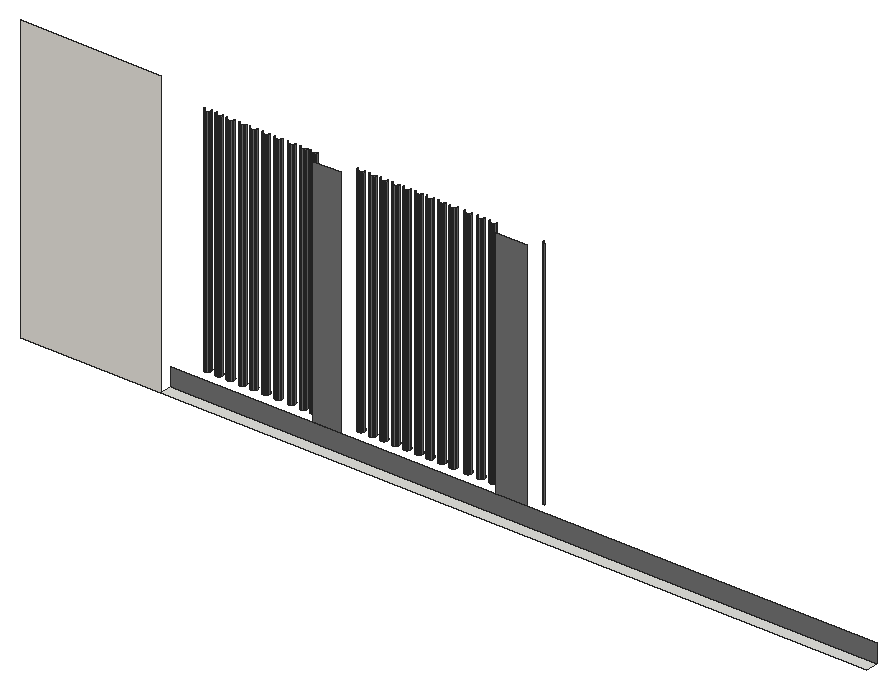
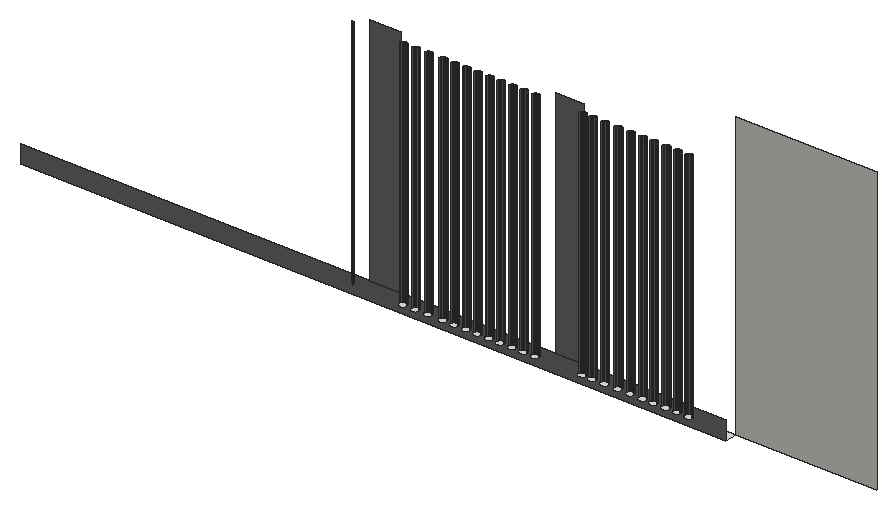
# SketchUp Ruby script. Lengths in inches.
U = 1.inch
M = Sketchup.active_model
def pt(a) = Geom::Point3d.new(a.map { |v| v * U })
def face(e, loops, mat)
  f = e.add_face(loops[0].map { |a| pt(a) })
  loops[1..].each { |l| e.add_face(l.map { |a| pt(a) }).erase! }
  f.material = f.back_material = mat if mat
  f
end
# faces: each face lists its corners as indices into pts; further lists are holes
def faces(e, pts, list, mat = nil) = list.each { |f| face(e, (f[0].is_a?(Array) ? f : [f]).map { |l| l.map { |i| pts[i] } }, mat) }
# xy, xz, yz: faces in a plane at the given z, y or x. An outline is a flat list of corners, or four numbers for a rectangle; further outlines are holes
def ring(l) = l.size == 4 ? [[l[0], l[1]], [l[2], l[1]], [l[2], l[3]], [l[0], l[3]]] : l.each_slice(2).to_a
def flat(e, list, mat, &to3) = list.each { |f| face(e, (f[0].is_a?(Array) ? f : [f]).map { |l| ring(l).map { |u, v| to3.(u, v) } }, mat) }
def xy(e, z, list, mat = nil) = flat(e, list, mat) { |x, y| [x, y, z] }
def xz(e, y, list, mat = nil) = flat(e, list, mat) { |x, z| [x, y, z] }
def yz(e, x, list, mat = nil) = flat(e, list, mat) { |y, z| [x, y, z] }
def lines(e, pts, list) = list.each { |a, b| e.add_line(pt(pts[a]), pt(pts[b])) }
# prism: a flat outline (further loops are holes) pulled along v
def prism(e, loops, v, mat = nil)
  f = face(e, loops, mat); d = Geom::Vector3d.new(v.map { |x| x * U })
  f.pushpull(f.normal.samedirection?(d) ? d.length : -d.length)
end
def box(e, o, s, mat = nil) = prism(e, [[o, [o[0] + s[0], o[1], o[2]], [o[0] + s[0], o[1] + s[1], o[2]], [o[0], o[1] + s[1], o[2]]]], [0, 0, s[2]], mat)
def at(x, y, z, deg = 0) = Geom::Transformation.translation(pt([x, y, z])) * Geom::Transformation.rotation(ORIGIN, Z_AXIS, deg.degrees)
def axes(o, x, y, z) = Geom::Transformation.new([*x, 0, *y, 0, *z, 0, *pt(o).to_a, 1])
def part(name) = M.definitions.add(name)
# library, detail: a bought-in or finely detailed component or shape, given as its bounding box
def library(name, o, s) = part(name).tap { |d| box(d.entities, o, s) }
def detail(e, o, s) = box(e.add_group.entities, o, s)
def put(e, d, t, mat = nil) = e.add_instance(d, t).tap { |i| i.material = mat if mat }
def group(e, t, mat = nil) = e.add_group.tap { |g| g.transformation = t; g.material = mat if mat }.entities
root = M.entities
M.materials.add("[Color M05]").color = [114, 114, 114]
M.materials.add("[Tile Travertine 2 inch]").color = [229, 225, 218]
xy(root,9,[[61.88,119.71,371.37,125.1875]])
xy(root,17.125,[[73.24,129.51,72.84,129.56,72.46,129.72,72.13,129.97,71.89,130.29,71.73,130.67,71.68,131.07,71.73,131.48,71.89,131.86,72.13,132.18,72.46,132.43,72.84,132.58,73.24,132.64,73.64,132.58,74.02,132.43,74.34,132.18,74.59,131.86,74.75,131.48,74.8,131.07,74.75,130.67,74.59,130.29,74.34,129.97,74.02,129.72,73.64,129.56],[78.3,129.51,77.9,129.56,77.52,129.72,77.2,129.97,76.95,130.29,76.79,130.67,76.74,131.07,76.79,131.48,76.95,131.86,77.2,132.18,77.52,132.43,77.9,132.58,78.3,132.64,78.71,132.58,79.08,132.43,79.41,132.18,79.66,131.86,79.8125,131.48,79.86,131.07,79.8125,130.67,79.66,130.29,79.41,129.97,79.08,129.72,78.71,129.56],[83.3,129.51,82.9,129.56,82.52,129.72,82.2,129.97,81.95,130.29,81.79,130.67,81.74,131.07,81.79,131.48,81.95,131.86,82.2,132.18,82.52,132.43,82.9,132.58,83.3,132.64,83.71,132.58,84.08,132.43,84.41,132.18,84.66,131.86,84.8125,131.48,84.86,131.07,84.8125,130.67,84.66,130.29,84.41,129.97,84.08,129.72,83.71,129.56],[88.61,129.51,88.21,129.56,87.83,129.72,87.51,129.97,87.26,130.29,87.11,130.67,87.05,131.07,87.11,131.48,87.26,131.86,87.51,132.18,87.83,132.43,88.21,132.58,88.61,132.64,89.02,132.58,89.4,132.43,89.72,132.18,89.97,131.86,90.125,131.48,90.18,131.07,90.125,130.67,89.97,130.29,89.72,129.97,89.4,129.72,89.02,129.56],[93.43,129.51,93.02,129.56,92.65,129.72,92.32,129.97,92.07,130.29,91.92,130.67,91.86,131.07,91.92,131.48,92.07,131.86,92.32,132.18,92.65,132.43,93.02,132.58,93.43,132.64,93.83,132.58,94.21,132.43,94.53,132.18,94.78,131.86,94.9375,131.48,94.99,131.07,94.9375,130.67,94.78,130.29,94.53,129.97,94.21,129.72,93.83,129.56],
  [98.93,129.51,98.52,129.56,98.15,129.72,97.82,129.97,97.57,130.29,97.42,130.67,97.36,131.07,97.42,131.48,97.57,131.86,97.82,132.18,98.15,132.43,98.52,132.58,98.93,132.64,99.33,132.58,99.71,132.43,100.03,132.18,100.28,131.86,100.4375,131.48,100.49,131.07,100.4375,130.67,100.28,130.29,100.03,129.97,99.71,129.72,99.33,129.56],[104.36,129.51,103.96,129.56,103.58,129.72,103.26,129.97,103.01,130.29,102.86,130.67,102.8,131.07,102.86,131.48,103.01,131.86,103.26,132.18,103.58,132.43,103.96,132.58,104.36,132.64,104.77,132.58,105.15,132.43,105.47,132.18,105.72,131.86,105.875,131.48,105.93,131.07,105.875,130.67,105.72,130.29,105.47,129.97,105.15,129.72,104.77,129.56],[110.11,129.51,109.71,129.56,109.33,129.72,109.01,129.97,108.76,130.29,108.61,130.67,108.55,131.07,108.61,131.48,108.76,131.86,109.01,132.18,109.33,132.43,109.71,132.58,110.11,132.64,110.52,132.58,110.9,132.43,111.22,132.18,111.47,131.86,111.625,131.48,111.68,131.07,111.625,130.67,111.47,130.29,111.22,129.97,110.9,129.72,110.52,129.56],[115.49,129.51,115.09,129.56,114.71,129.72,114.38,129.97,114.14,130.29,113.98,130.67,113.93,131.07,113.98,131.48,114.14,131.86,114.38,132.18,114.71,132.43,115.09,132.58,115.49,132.64,115.89,132.58,116.27,132.43,116.59,132.18,116.84,131.86,117,131.48,117.05,131.07,117,130.67,116.84,130.29,116.59,129.97,116.27,129.72,115.89,129.56],[119.99,129.51,119.59,129.56,119.21,129.72,118.88,129.97,118.64,130.29,118.48,130.67,118.43,131.07,118.48,131.48,118.64,131.86,118.88,132.18,119.21,132.43,119.59,132.58,119.99,132.64,120.39,132.58,120.77,132.43,121.09,132.18,121.34,131.86,121.5,131.48,121.55,131.07,121.5,130.67,121.34,130.29,121.09,129.97,120.77,129.72,120.39,129.56],
  [140.68,129.51,140.27,129.56,139.9,129.72,139.57,129.97,139.32,130.29,139.17,130.67,139.11,131.07,139.17,131.48,139.32,131.86,139.57,132.18,139.9,132.43,140.27,132.58,140.68,132.64,141.08,132.58,141.46,132.43,141.78,132.18,142.03,131.86,142.1875,131.48,142.24,131.07,142.1875,130.67,142.03,130.29,141.78,129.97,141.46,129.72,141.08,129.56],[145.74,129.51,145.34,129.56,144.96,129.72,144.63,129.97,144.39,130.29,144.23,130.67,144.18,131.07,144.23,131.48,144.39,131.86,144.63,132.18,144.96,132.43,145.34,132.58,145.74,132.64,146.14,132.58,146.52,132.43,146.84,132.18,147.09,131.86,147.25,131.48,147.3,131.07,147.25,130.67,147.09,130.29,146.84,129.97,146.52,129.72,146.14,129.56],[150.8,129.51,150.4,129.56,150.02,129.72,149.7,129.97,149.45,130.29,149.29,130.67,149.24,131.07,149.29,131.48,149.45,131.86,149.7,132.18,150.02,132.43,150.4,132.58,150.8,132.64,151.21,132.58,151.58,132.43,151.91,132.18,152.16,131.86,152.3125,131.48,152.36,131.07,152.3125,130.67,152.16,130.29,151.91,129.97,151.58,129.72,151.21,129.56],[155.86,129.51,155.46,129.56,155.08,129.72,154.76,129.97,154.51,130.29,154.36,130.67,154.3,131.07,154.36,131.48,154.51,131.86,154.76,132.18,155.08,132.43,155.46,132.58,155.86,132.64,156.27,132.58,156.65,132.43,156.97,132.18,157.22,131.86,157.375,131.48,157.43,131.07,157.375,130.67,157.22,130.29,156.97,129.97,156.65,129.72,156.27,129.56],[160.93,129.51,160.52,129.56,160.15,129.72,159.82,129.97,159.57,130.29,159.42,130.67,159.36,131.07,159.42,131.48,159.57,131.86,159.82,132.18,160.15,132.43,160.52,132.58,160.93,132.64,161.33,132.58,161.71,132.43,162.03,132.18,162.28,131.86,162.4375,131.48,162.49,131.07,162.4375,130.67,162.28,130.29,162.03,129.97,161.71,129.72,161.33,129.56],
  [165.99,129.51,165.59,129.56,165.21,129.72,164.88,129.97,164.64,130.29,164.48,130.67,164.43,131.07,164.48,131.48,164.64,131.86,164.88,132.18,165.21,132.43,165.59,132.58,165.99,132.64,166.39,132.58,166.77,132.43,167.09,132.18,167.34,131.86,167.5,131.48,167.55,131.07,167.5,130.67,167.34,130.29,167.09,129.97,166.77,129.72,166.39,129.56],[171.05,129.51,170.65,129.56,170.27,129.72,169.95,129.97,169.7,130.29,169.54,130.67,169.49,131.07,169.54,131.48,169.7,131.86,169.95,132.18,170.27,132.43,170.65,132.58,171.05,132.64,171.46,132.58,171.83,132.43,172.16,132.18,172.41,131.86,172.5625,131.48,172.61,131.07,172.5625,130.67,172.41,130.29,172.16,129.97,171.83,129.72,171.46,129.56],[176.11,129.51,175.71,129.56,175.33,129.72,175.01,129.97,174.76,130.29,174.61,130.67,174.55,131.07,174.61,131.48,174.76,131.86,175.01,132.18,175.33,132.43,175.71,132.58,176.11,132.64,176.52,132.58,176.9,132.43,177.22,132.18,177.47,131.86,177.625,131.48,177.68,131.07,177.625,130.67,177.47,130.29,177.22,129.97,176.9,129.72,176.52,129.56],[181.18,129.51,180.77,129.56,180.4,129.72,180.07,129.97,179.82,130.29,179.67,130.67,179.61,131.07,179.67,131.48,179.82,131.86,180.07,132.18,180.4,132.43,180.77,132.58,181.18,132.64,181.58,132.58,181.96,132.43,182.28,132.18,182.53,131.86,182.6875,131.48,182.74,131.07,182.6875,130.67,182.53,130.29,182.28,129.97,181.96,129.72,181.58,129.56],[187.68,129.51,187.27,129.56,186.9,129.72,186.57,129.97,186.32,130.29,186.17,130.67,186.11,131.07,186.17,131.48,186.32,131.86,186.57,132.18,186.9,132.43,187.27,132.58,187.68,132.64,188.08,132.58,188.46,132.43,188.78,132.18,189.03,131.86,189.1875,131.48,189.24,131.07,189.1875,130.67,189.03,130.29,188.78,129.97,188.46,129.72,188.08,129.56],
  [193.18,129.51,192.77,129.56,192.4,129.72,192.07,129.97,191.82,130.29,191.67,130.67,191.61,131.07,191.67,131.48,191.82,131.86,192.07,132.18,192.4,132.43,192.77,132.58,193.18,132.64,193.58,132.58,193.96,132.43,194.28,132.18,194.53,131.86,194.6875,131.48,194.74,131.07,194.6875,130.67,194.53,130.29,194.28,129.97,193.96,129.72,193.58,129.56],[198.68,129.51,198.27,129.56,197.9,129.72,197.57,129.97,197.32,130.29,197.17,130.67,197.11,131.07,197.17,131.48,197.32,131.86,197.57,132.18,197.9,132.43,198.27,132.58,198.68,132.64,199.08,132.58,199.46,132.43,199.78,132.18,200.03,131.86,200.1875,131.48,200.24,131.07,200.1875,130.67,200.03,130.29,199.78,129.97,199.46,129.72,199.08,129.56]])
xz(root,119.71,[[0,9,61.88,133.9375]],"[Tile Travertine 2 inch]")
xz(root,125.1875,[[61.88,9,371.37,17.125],[124.17,17.125,136.24,119.59],[204.36,17.125,217.93,119.59]],"[Color M05]")
p = [[72.84,129.56,17.125],[73.24,129.51,17.125],[73.24,129.51,119.59],[72.84,129.56,119.59],[73.64,129.56,17.125],[73.64,129.56,119.59],
  [77.9,129.56,17.125],[78.3,129.51,17.125],[78.3,129.51,119.59],[77.9,129.56,119.59],[78.71,129.56,17.125],[78.71,129.56,119.59],
  [82.9,129.56,17.125],[83.3,129.51,17.125],[83.3,129.51,119.59],[82.9,129.56,119.59],[83.71,129.56,17.125],[83.71,129.56,119.59],
  [88.21,129.56,17.125],[88.61,129.51,17.125],[88.61,129.51,119.59],[88.21,129.56,119.59],[89.02,129.56,17.125],[89.02,129.56,119.59],
  [93.02,129.56,17.125],[93.43,129.51,17.125],[93.43,129.51,119.59],[93.02,129.56,119.59],[93.83,129.56,17.125],[93.83,129.56,119.59],
  [98.52,129.56,17.125],[98.93,129.51,17.125],[98.93,129.51,119.59],[98.52,129.56,119.59],[99.33,129.56,17.125],[99.33,129.56,119.59],
  [103.96,129.56,17.125],[104.36,129.51,17.125],[104.36,129.51,119.59],[103.96,129.56,119.59],[104.77,129.56,17.125],[104.77,129.56,119.59],
  [109.71,129.56,17.125],[110.11,129.51,17.125],[110.11,129.51,119.59],[109.71,129.56,119.59],[110.52,129.56,17.125],[110.52,129.56,119.59],
  [115.09,129.56,17.125],[115.49,129.51,17.125],[115.49,129.51,119.59],[115.09,129.56,119.59],[115.89,129.56,17.125],[115.89,129.56,119.59],
  [119.59,129.56,17.125],[119.99,129.51,17.125],[119.99,129.51,119.59],[119.59,129.56,119.59],[120.39,129.56,17.125],[120.39,129.56,119.59],
  [140.27,129.56,17.125],[140.68,129.51,17.125],[140.68,129.51,119.59],[140.27,129.56,119.59],[141.08,129.56,17.125],[141.08,129.56,119.59],
  [145.34,129.56,17.125],[145.74,129.51,17.125],[145.74,129.51,119.59],[145.34,129.56,119.59],[146.14,129.56,17.125],[146.14,129.56,119.59],
  [150.4,129.56,17.125],[150.8,129.51,17.125],[150.8,129.51,119.59],[150.4,129.56,119.59],[151.21,129.56,17.125],[151.21,129.56,119.59],
  [155.46,129.56,17.125],[155.86,129.51,17.125],[155.86,129.51,119.59],[155.46,129.56,119.59],[156.27,129.56,17.125],[156.27,129.56,119.59],
  [160.52,129.56,17.125],[160.93,129.51,17.125],[160.93,129.51,119.59],[160.52,129.56,119.59],[161.33,129.56,17.125],[161.33,129.56,119.59],
  [165.59,129.56,17.125],[165.99,129.51,17.125],[165.99,129.51,119.59],[165.59,129.56,119.59],[166.39,129.56,17.125],[166.39,129.56,119.59],
  [170.65,129.56,17.125],[171.05,129.51,17.125],[171.05,129.51,119.59],[170.65,129.56,119.59],[171.46,129.56,17.125],[171.46,129.56,119.59],
  [175.71,129.56,17.125],[176.11,129.51,17.125],[176.11,129.51,119.59],[175.71,129.56,119.59],[176.52,129.56,17.125],[176.52,129.56,119.59],
  [180.77,129.56,17.125],[181.18,129.51,17.125],[181.18,129.51,119.59],[180.77,129.56,119.59],[181.58,129.56,17.125],[181.58,129.56,119.59],
  [187.27,129.56,17.125],[187.68,129.51,17.125],[187.68,129.51,119.59],[187.27,129.56,119.59],[188.08,129.56,17.125],[188.08,129.56,119.59],
  [192.77,129.56,17.125],[193.18,129.51,17.125],[193.18,129.51,119.59],[192.77,129.56,119.59],[193.58,129.56,17.125],[193.58,129.56,119.59],
  [198.27,129.56,17.125],[198.68,129.51,17.125],[198.68,129.51,119.59],[198.27,129.56,119.59],[199.08,129.56,17.125],[199.08,129.56,119.59],
  [221.84,129.56,17.125],[222.24,129.51,17.125],[222.24,129.51,119.59],[221.84,129.56,119.59],[72.46,129.72,17.125],[72.46,129.72,119.59],
  [74.02,129.72,17.125],[74.02,129.72,119.59],[77.52,129.72,17.125],[77.52,129.72,119.59],[79.08,129.72,17.125],[79.08,129.72,119.59],
  [82.52,129.72,17.125],[82.52,129.72,119.59],[84.08,129.72,17.125],[84.08,129.72,119.59],[87.83,129.72,17.125],[87.83,129.72,119.59],
  [89.4,129.72,17.125],[89.4,129.72,119.59],[92.65,129.72,17.125],[92.65,129.72,119.59],[94.21,129.72,17.125],[94.21,129.72,119.59],
  [98.15,129.72,17.125],[98.15,129.72,119.59],[99.71,129.72,17.125],[99.71,129.72,119.59],[103.58,129.72,17.125],[103.58,129.72,119.59],
  [105.15,129.72,17.125],[105.15,129.72,119.59],[109.33,129.72,17.125],[109.33,129.72,119.59],[110.9,129.72,17.125],[110.9,129.72,119.59],
  [114.71,129.72,17.125],[114.71,129.72,119.59],[116.27,129.72,17.125],[116.27,129.72,119.59],[119.21,129.72,17.125],[119.21,129.72,119.59],
  [120.77,129.72,17.125],[120.77,129.72,119.59],[139.9,129.72,17.125],[139.9,129.72,119.59],[141.46,129.72,17.125],[141.46,129.72,119.59],
  [144.96,129.72,17.125],[144.96,129.72,119.59],[146.52,129.72,17.125],[146.52,129.72,119.59],[150.02,129.72,17.125],[150.02,129.72,119.59],
  [151.58,129.72,17.125],[151.58,129.72,119.59],[155.08,129.72,17.125],[155.08,129.72,119.59],[156.65,129.72,17.125],[156.65,129.72,119.59],
  [160.15,129.72,17.125],[160.15,129.72,119.59],[161.71,129.72,17.125],[161.71,129.72,119.59],[165.21,129.72,17.125],[165.21,129.72,119.59],
  [166.77,129.72,17.125],[166.77,129.72,119.59],[170.27,129.72,17.125],[170.27,129.72,119.59],[171.83,129.72,17.125],[171.83,129.72,119.59],
  [175.33,129.72,17.125],[175.33,129.72,119.59],[176.9,129.72,17.125],[176.9,129.72,119.59],[180.4,129.72,17.125],[180.4,129.72,119.59],
  [181.96,129.72,17.125],[181.96,129.72,119.59],[186.9,129.72,17.125],[186.9,129.72,119.59],[188.46,129.72,17.125],[188.46,129.72,119.59],
  [192.4,129.72,17.125],[192.4,129.72,119.59],[193.96,129.72,17.125],[193.96,129.72,119.59],[197.9,129.72,17.125],[197.9,129.72,119.59],
  [199.46,129.72,17.125],[199.46,129.72,119.59],[221.46,129.72,17.125],[221.46,129.72,119.59],[72.13,129.97,17.125],[72.13,129.97,119.59],
  [74.34,129.97,17.125],[74.34,129.97,119.59],[77.2,129.97,17.125],[77.2,129.97,119.59],[79.41,129.97,17.125],[79.41,129.97,119.59],
  [82.2,129.97,17.125],[82.2,129.97,119.59],[84.41,129.97,17.125],[84.41,129.97,119.59],[87.51,129.97,17.125],[87.51,129.97,119.59],
  [89.72,129.97,17.125],[89.72,129.97,119.59],[92.32,129.97,17.125],[92.32,129.97,119.59],[94.53,129.97,17.125],[94.53,129.97,119.59],
  [97.82,129.97,17.125],[97.82,129.97,119.59],[100.03,129.97,17.125],[100.03,129.97,119.59],[103.26,129.97,17.125],[103.26,129.97,119.59],
  [105.47,129.97,17.125],[105.47,129.97,119.59],[109.01,129.97,17.125],[109.01,129.97,119.59],[111.22,129.97,17.125],[111.22,129.97,119.59],
  [114.38,129.97,17.125],[114.38,129.97,119.59],[116.59,129.97,17.125],[116.59,129.97,119.59],[118.88,129.97,17.125],[118.88,129.97,119.59],
  [121.09,129.97,17.125],[121.09,129.97,119.59],[139.57,129.97,17.125],[139.57,129.97,119.59],[141.78,129.97,17.125],[141.78,129.97,119.59],
  [144.63,129.97,17.125],[144.63,129.97,119.59],[146.84,129.97,17.125],[146.84,129.97,119.59],[149.7,129.97,17.125],[149.7,129.97,119.59],
  [151.91,129.97,17.125],[151.91,129.97,119.59],[154.76,129.97,17.125],[154.76,129.97,119.59],[156.97,129.97,17.125],[156.97,129.97,119.59],
  [159.82,129.97,17.125],[159.82,129.97,119.59],[162.03,129.97,17.125],[162.03,129.97,119.59],[164.88,129.97,17.125],[164.88,129.97,119.59],
  [167.09,129.97,17.125],[167.09,129.97,119.59],[169.95,129.97,17.125],[169.95,129.97,119.59],[172.16,129.97,17.125],[172.16,129.97,119.59],
  [175.01,129.97,17.125],[175.01,129.97,119.59],[177.22,129.97,17.125],[177.22,129.97,119.59],[180.07,129.97,17.125],[180.07,129.97,119.59],
  [182.28,129.97,17.125],[182.28,129.97,119.59],[186.57,129.97,17.125],[186.57,129.97,119.59],[188.78,129.97,17.125],[188.78,129.97,119.59],
  [192.07,129.97,17.125],[192.07,129.97,119.59],[194.28,129.97,17.125],[194.28,129.97,119.59],[197.57,129.97,17.125],[197.57,129.97,119.59],
  [199.78,129.97,17.125],[199.78,129.97,119.59],[221.13,129.97,17.125],[221.13,129.97,119.59],[71.89,130.29,17.125],[71.89,130.29,119.59],
  [74.59,130.29,17.125],[74.59,130.29,119.59],[76.95,130.29,17.125],[76.95,130.29,119.59],[79.66,130.29,17.125],[79.66,130.29,119.59],
  [81.95,130.29,17.125],[81.95,130.29,119.59],[84.66,130.29,17.125],[84.66,130.29,119.59],[87.26,130.29,17.125],[87.26,130.29,119.59],
  [89.97,130.29,17.125],[89.97,130.29,119.59],[92.07,130.29,17.125],[92.07,130.29,119.59],[94.78,130.29,17.125],[94.78,130.29,119.59],
  [97.57,130.29,17.125],[97.57,130.29,119.59],[100.28,130.29,17.125],[100.28,130.29,119.59],[103.01,130.29,17.125],[103.01,130.29,119.59],
  [105.72,130.29,17.125],[105.72,130.29,119.59],[108.76,130.29,17.125],[108.76,130.29,119.59],[111.47,130.29,17.125],[111.47,130.29,119.59],
  [114.14,130.29,17.125],[114.14,130.29,119.59],[116.84,130.29,17.125],[116.84,130.29,119.59],[118.64,130.29,17.125],[118.64,130.29,119.59],
  [121.34,130.29,17.125],[121.34,130.29,119.59],[139.32,130.29,17.125],[139.32,130.29,119.59],[142.03,130.29,17.125],[142.03,130.29,119.59],
  [144.39,130.29,17.125],[144.39,130.29,119.59],[147.09,130.29,17.125],[147.09,130.29,119.59],[149.45,130.29,17.125],[149.45,130.29,119.59],
  [152.16,130.29,17.125],[152.16,130.29,119.59],[154.51,130.29,17.125],[154.51,130.29,119.59],[157.22,130.29,17.125],[157.22,130.29,119.59],
  [159.57,130.29,17.125],[159.57,130.29,119.59],[162.28,130.29,17.125],[162.28,130.29,119.59],[164.64,130.29,17.125],[164.64,130.29,119.59],
  [167.34,130.29,17.125],[167.34,130.29,119.59],[169.7,130.29,17.125],[169.7,130.29,119.59],[172.41,130.29,17.125],[172.41,130.29,119.59],
  [174.76,130.29,17.125],[174.76,130.29,119.59],[177.47,130.29,17.125],[177.47,130.29,119.59],[179.82,130.29,17.125],[179.82,130.29,119.59],
  [182.53,130.29,17.125],[182.53,130.29,119.59],[186.32,130.29,17.125],[186.32,130.29,119.59],[189.03,130.29,17.125],[189.03,130.29,119.59],
  [191.82,130.29,17.125],[191.82,130.29,119.59],[194.53,130.29,17.125],[194.53,130.29,119.59],[197.32,130.29,17.125],[197.32,130.29,119.59],
  [200.03,130.29,17.125],[200.03,130.29,119.59],[220.89,130.29,17.125],[220.89,130.29,119.59],[71.73,130.67,17.125],[71.73,130.67,119.59],
  [74.75,130.67,17.125],[74.75,130.67,119.59],[76.79,130.67,17.125],[76.79,130.67,119.59],[79.8125,130.67,17.125],[79.8125,130.67,119.59],
  [81.79,130.67,17.125],[81.79,130.67,119.59],[84.8125,130.67,17.125],[84.8125,130.67,119.59],[87.11,130.67,17.125],[87.11,130.67,119.59],
  [90.125,130.67,17.125],[90.125,130.67,119.59],[91.92,130.67,17.125],[91.92,130.67,119.59],[94.9375,130.67,17.125],[94.9375,130.67,119.59],
  [97.42,130.67,17.125],[97.42,130.67,119.59],[100.4375,130.67,17.125],[100.4375,130.67,119.59],[102.86,130.67,17.125],[102.86,130.67,119.59],
  [105.875,130.67,17.125],[105.875,130.67,119.59],[108.61,130.67,17.125],[108.61,130.67,119.59],[111.625,130.67,17.125],[111.625,130.67,119.59],
  [113.98,130.67,17.125],[113.98,130.67,119.59],[117,130.67,17.125],[117,130.67,119.59],[118.48,130.67,17.125],[118.48,130.67,119.59],
  [121.5,130.67,17.125],[121.5,130.67,119.59],[139.17,130.67,17.125],[139.17,130.67,119.59],[142.1875,130.67,17.125],[142.1875,130.67,119.59],
  [144.23,130.67,17.125],[144.23,130.67,119.59],[147.25,130.67,17.125],[147.25,130.67,119.59],[149.29,130.67,17.125],[149.29,130.67,119.59],
  [152.3125,130.67,17.125],[152.3125,130.67,119.59],[154.36,130.67,17.125],[154.36,130.67,119.59],[157.375,130.67,17.125],[157.375,130.67,119.59],
  [159.42,130.67,17.125],[159.42,130.67,119.59],[162.4375,130.67,17.125],[162.4375,130.67,119.59],[164.48,130.67,17.125],[164.48,130.67,119.59],
  [167.5,130.67,17.125],[167.5,130.67,119.59],[169.54,130.67,17.125],[169.54,130.67,119.59],[172.5625,130.67,17.125],[172.5625,130.67,119.59],
  [174.61,130.67,17.125],[174.61,130.67,119.59],[177.625,130.67,17.125],[177.625,130.67,119.59],[179.67,130.67,17.125],[179.67,130.67,119.59],
  [182.6875,130.67,17.125],[182.6875,130.67,119.59],[186.17,130.67,17.125],[186.17,130.67,119.59],[189.1875,130.67,17.125],[189.1875,130.67,119.59],
  [191.67,130.67,17.125],[191.67,130.67,119.59],[194.6875,130.67,17.125],[194.6875,130.67,119.59],[197.17,130.67,17.125],[197.17,130.67,119.59],
  [200.1875,130.67,17.125],[200.1875,130.67,119.59],[220.73,130.67,17.125],[220.73,130.67,119.59],[71.68,131.07,17.125],[71.68,131.07,119.59],
  [74.8,131.07,17.125],[74.8,131.07,119.59],[76.74,131.07,17.125],[76.74,131.07,119.59],[79.86,131.07,17.125],[79.86,131.07,119.59],
  [81.74,131.07,17.125],[81.74,131.07,119.59],[84.86,131.07,17.125],[84.86,131.07,119.59],[87.05,131.07,17.125],[87.05,131.07,119.59],
  [90.18,131.07,17.125],[90.18,131.07,119.59],[91.86,131.07,17.125],[91.86,131.07,119.59],[94.99,131.07,17.125],[94.99,131.07,119.59],
  [97.36,131.07,17.125],[97.36,131.07,119.59],[100.49,131.07,17.125],[100.49,131.07,119.59],[102.8,131.07,17.125],[102.8,131.07,119.59],
  [105.93,131.07,17.125],[105.93,131.07,119.59],[108.55,131.07,17.125],[108.55,131.07,119.59],[111.68,131.07,17.125],[111.68,131.07,119.59],
  [113.93,131.07,17.125],[113.93,131.07,119.59],[117.05,131.07,17.125],[117.05,131.07,119.59],[118.43,131.07,17.125],[118.43,131.07,119.59],
  [121.55,131.07,17.125],[121.55,131.07,119.59],[139.11,131.07,17.125],[139.11,131.07,119.59],[142.24,131.07,17.125],[142.24,131.07,119.59],
  [144.18,131.07,17.125],[144.18,131.07,119.59],[147.3,131.07,17.125],[147.3,131.07,119.59],[149.24,131.07,17.125],[149.24,131.07,119.59],
  [152.36,131.07,17.125],[152.36,131.07,119.59],[154.3,131.07,17.125],[154.3,131.07,119.59],[157.43,131.07,17.125],[157.43,131.07,119.59],
  [159.36,131.07,17.125],[159.36,131.07,119.59],[162.49,131.07,17.125],[162.49,131.07,119.59],[164.43,131.07,17.125],[164.43,131.07,119.59],
  [167.55,131.07,17.125],[167.55,131.07,119.59],[169.49,131.07,17.125],[169.49,131.07,119.59],[172.61,131.07,17.125],[172.61,131.07,119.59],
  [174.55,131.07,17.125],[174.55,131.07,119.59],[177.68,131.07,17.125],[177.68,131.07,119.59],[179.61,131.07,17.125],[179.61,131.07,119.59],
  [182.74,131.07,17.125],[182.74,131.07,119.59],[186.11,131.07,17.125],[186.11,131.07,119.59],[189.24,131.07,17.125],[189.24,131.07,119.59],
  [191.61,131.07,17.125],[191.61,131.07,119.59],[194.74,131.07,17.125],[194.74,131.07,119.59],[197.11,131.07,17.125],[197.11,131.07,119.59],
  [200.24,131.07,17.125],[200.24,131.07,119.59],[220.68,131.07,17.125],[220.68,131.07,119.59],[71.73,131.48,17.125],[71.73,131.48,119.59],
  [74.75,131.48,17.125],[74.75,131.48,119.59],[76.79,131.48,17.125],[76.79,131.48,119.59]]
faces(root,p,[[0,1,2,3],[1,4,5,2],[6,7,8,9],[7,10,11,8],[12,13,14,15],[13,16,17,14],[18,19,20,21],[19,22,23,20],
  [24,25,26,27],[25,28,29,26],[30,31,32,33],[31,34,35,32],[36,37,38,39],[37,40,41,38],[42,43,44,45],[43,46,47,44],
  [48,49,50,51],[49,52,53,50],[54,55,56,57],[55,58,59,56],[60,61,62,63],[61,64,65,62],[66,67,68,69],[67,70,71,68],
  [72,73,74,75],[73,76,77,74],[78,79,80,81],[79,82,83,80],[84,85,86,87],[85,88,89,86],[90,91,92,93],[91,94,95,92],
  [96,97,98,99],[97,100,101,98],[102,103,104,105],[103,106,107,104],[108,109,110,111],[109,112,113,110],[114,115,116,117],[115,118,119,116],
  [120,121,122,123],[121,124,125,122],[126,127,128,129],[127,130,131,128],[132,133,134,135],[136,0,3,137],[4,138,139,5],[140,6,9,141],
  [10,142,143,11],[144,12,15,145],[16,146,147,17],[148,18,21,149],[22,150,151,23],[152,24,27,153],[28,154,155,29],[156,30,33,157],
  [34,158,159,35],[160,36,39,161],[40,162,163,41],[164,42,45,165],[46,166,167,47],[168,48,51,169],[52,170,171,53],[172,54,57,173],
  [58,174,175,59],[176,60,63,177],[64,178,179,65],[180,66,69,181],[70,182,183,71],[184,72,75,185],[76,186,187,77],[188,78,81,189],
  [82,190,191,83],[192,84,87,193],[88,194,195,89],[196,90,93,197],[94,198,199,95],[200,96,99,201],[100,202,203,101],[204,102,105,205],
  [106,206,207,107],[208,108,111,209],[112,210,211,113],[212,114,117,213],[118,214,215,119],[216,120,123,217],[124,218,219,125],[220,126,129,221],
  [130,222,223,131],[224,132,135,225],[226,136,137,227],[138,228,229,139],[230,140,141,231],[142,232,233,143],[234,144,145,235],[146,236,237,147],
  [238,148,149,239],[150,240,241,151],[242,152,153,243],[154,244,245,155],[246,156,157,247],[158,248,249,159],[250,160,161,251],[162,252,253,163],
  [254,164,165,255],[166,256,257,167],[258,168,169,259],[170,260,261,171],[262,172,173,263],[174,264,265,175],[266,176,177,267],[178,268,269,179],
  [270,180,181,271],[182,272,273,183],[274,184,185,275],[186,276,277,187],[278,188,189,279],[190,280,281,191],[282,192,193,283],[194,284,285,195],
  [286,196,197,287],[198,288,289,199],[290,200,201,291],[202,292,293,203],[294,204,205,295],[206,296,297,207],[298,208,209,299],[210,300,301,211],
  [302,212,213,303],[214,304,305,215],[306,216,217,307],[218,308,309,219],[310,220,221,311],[222,312,313,223],[314,224,225,315],[316,226,227,317],
  [228,318,319,229],[320,230,231,321],[232,322,323,233],[324,234,235,325],[236,326,327,237],[328,238,239,329],[240,330,331,241],[332,242,243,333],
  [244,334,335,245],[336,246,247,337],[248,338,339,249],[340,250,251,341],[252,342,343,253],[344,254,255,345],[256,346,347,257],[348,258,259,349],
  [260,350,351,261],[352,262,263,353],[264,354,355,265],[356,266,267,357],[268,358,359,269],[360,270,271,361],[272,362,363,273],[364,274,275,365],
  [276,366,367,277],[368,278,279,369],[280,370,371,281],[372,282,283,373],[284,374,375,285],[376,286,287,377],[288,378,379,289],[380,290,291,381],
  [292,382,383,293],[384,294,295,385],[296,386,387,297],[388,298,299,389],[300,390,391,301],[392,302,303,393],[304,394,395,305],[396,306,307,397],
  [308,398,399,309],[400,310,311,401],[312,402,403,313],[404,314,315,405],[406,316,317,407],[318,408,409,319],[410,320,321,411],[322,412,413,323],
  [414,324,325,415],[326,416,417,327],[418,328,329,419],[330,420,421,331],[422,332,333,423],[334,424,425,335],[426,336,337,427],[338,428,429,339],
  [430,340,341,431],[342,432,433,343],[434,344,345,435],[346,436,437,347],[438,348,349,439],[350,440,441,351],[442,352,353,443],[354,444,445,355],
  [446,356,357,447],[358,448,449,359],[450,360,361,451],[362,452,453,363],[454,364,365,455],[366,456,457,367],[458,368,369,459],[370,460,461,371],
  [462,372,373,463],[374,464,465,375],[466,376,377,467],[378,468,469,379],[470,380,381,471],[382,472,473,383],[474,384,385,475],[386,476,477,387],
  [478,388,389,479],[390,480,481,391],[482,392,393,483],[394,484,485,395],[486,396,397,487],[398,488,489,399],[490,400,401,491],[402,492,493,403],
  [494,404,405,495],[496,406,407,497],[408,498,499,409],[500,410,411,501],[412,502,503,413],[504,414,415,505],[416,506,507,417],[508,418,419,509],
  [420,510,511,421],[512,422,423,513],[424,514,515,425],[516,426,427,517],[428,518,519,429],[520,430,431,521],[432,522,523,433],[524,434,435,525],
  [436,526,527,437],[528,438,439,529],[440,530,531,441],[532,442,443,533],[444,534,535,445],[536,446,447,537],[448,538,539,449],[540,450,451,541],
  [452,542,543,453],[544,454,455,545],[456,546,547,457],[548,458,459,549],[460,550,551,461],[552,462,463,553],[464,554,555,465],[556,466,467,557],
  [468,558,559,469],[560,470,471,561],[472,562,563,473],[564,474,475,565],[476,566,567,477],[568,478,479,569],[480,570,571,481],[572,482,483,573],
  [484,574,575,485],[576,486,487,577],[488,578,579,489],[580,490,491,581],[492,582,583,493],[584,494,495,585],[586,496,497,587],[498,588,589,499],
  [590,500,501,591]],"[Color M05]")
